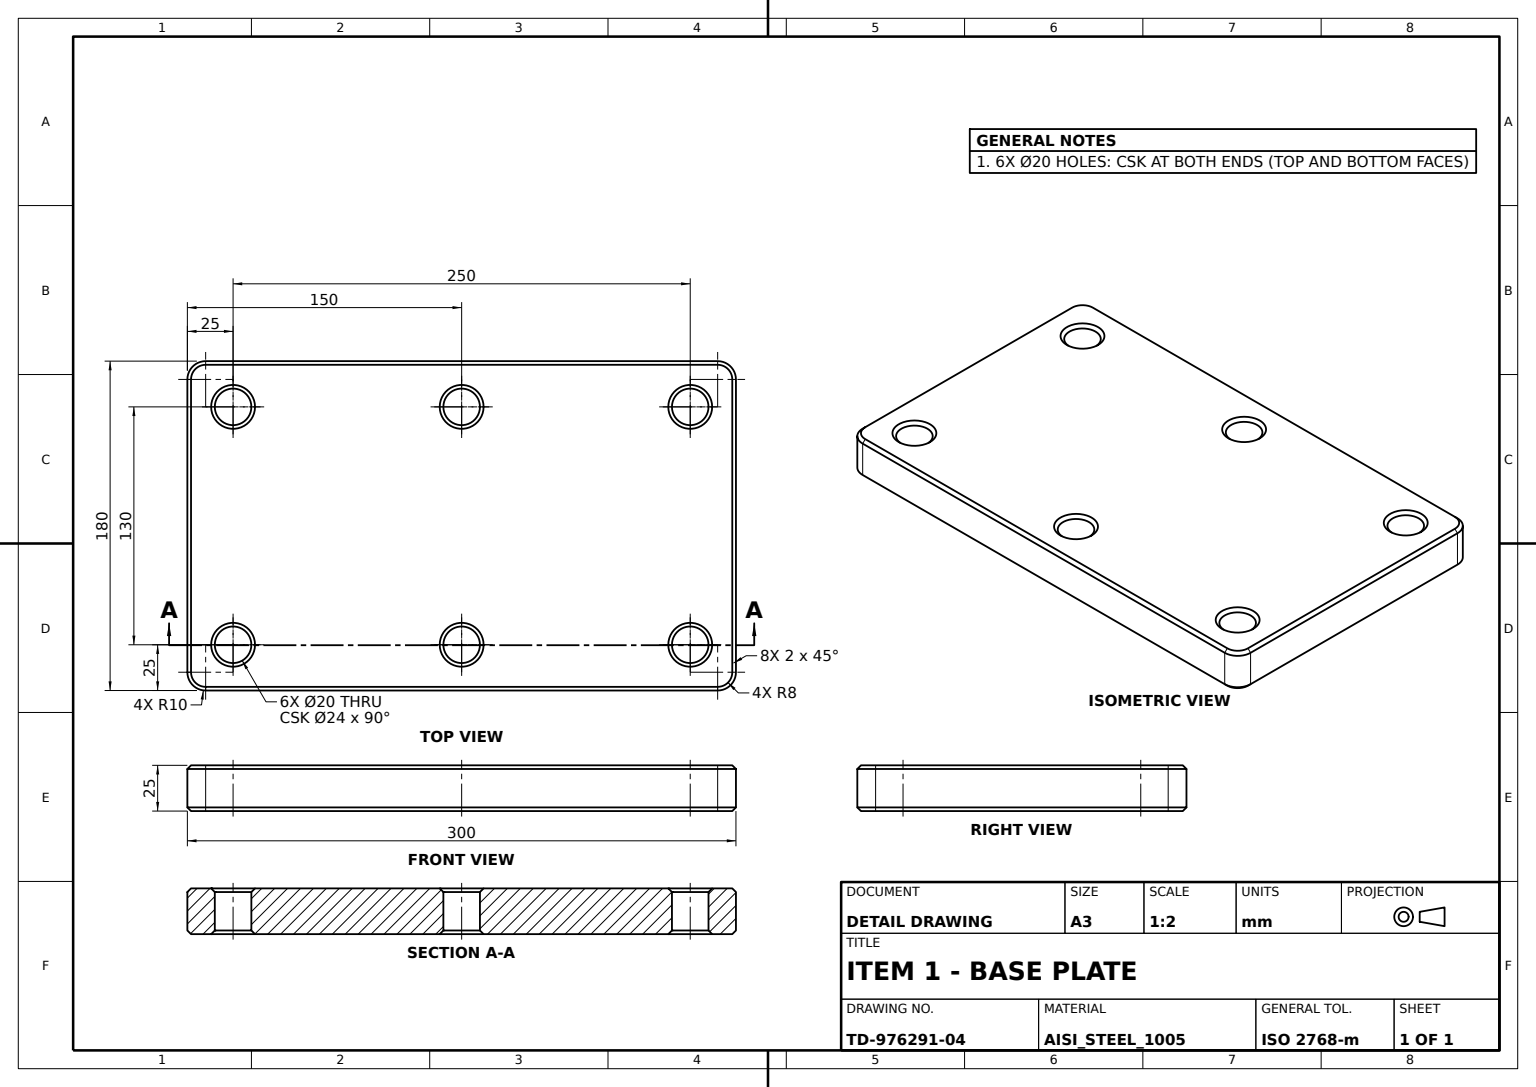
ISO-10303-21;
HEADER;
FILE_DESCRIPTION((''),'2;1');
FILE_NAME('','',(''),(''),'','','');
FILE_SCHEMA(('AUTOMOTIVE_DESIGN'));
ENDSEC;
DATA;
#1=APPLICATION_CONTEXT('');
#2=PRODUCT_CONTEXT('',#1,'mechanical');
#3=PRODUCT('','','',(#2));
#4=PRODUCT_DEFINITION_FORMATION('','',#3);
#5=PRODUCT_DEFINITION_CONTEXT('',#1,'design');
#6=PRODUCT_DEFINITION('','',#4,#5);
#7=PRODUCT_DEFINITION_SHAPE('','',#6);
#8=(LENGTH_UNIT()NAMED_UNIT(*)SI_UNIT(.MILLI.,.METRE.));
#9=(NAMED_UNIT(*)PLANE_ANGLE_UNIT()SI_UNIT($,.RADIAN.));
#10=(NAMED_UNIT(*)SI_UNIT($,.STERADIAN.)SOLID_ANGLE_UNIT());
#11=UNCERTAINTY_MEASURE_WITH_UNIT(LENGTH_MEASURE(0.005),#8,'distance_accuracy_value','');
#12=(GEOMETRIC_REPRESENTATION_CONTEXT(3)GLOBAL_UNCERTAINTY_ASSIGNED_CONTEXT((#11))GLOBAL_UNIT_ASSIGNED_CONTEXT((#8,#9,#10))REPRESENTATION_CONTEXT('',''));
#13=CARTESIAN_POINT('',(135.,65.,23.));
#14=VERTEX_POINT('',#13);
#15=CARTESIAN_POINT('',(125.,65.,23.));
#16=DIRECTION('',(0.,0.,1.));
#17=DIRECTION('',(1.,0.,0.));
#18=AXIS2_PLACEMENT_3D('',#15,#16,#17);
#19=CIRCLE('',#18,10.);
#20=EDGE_CURVE('',#14,#14,#19,.T.);
#21=ORIENTED_EDGE('',*,*,#20,.T.);
#22=EDGE_LOOP('',(#21));
#23=FACE_BOUND('',#22,.T.);
#24=CARTESIAN_POINT('',(135.,65.,2.));
#25=VERTEX_POINT('',#24);
#26=CARTESIAN_POINT('',(125.,65.,2.));
#27=AXIS2_PLACEMENT_3D('',#26,#16,#17);
#28=CIRCLE('',#27,10.);
#29=EDGE_CURVE('',#25,#25,#28,.F.);
#30=ORIENTED_EDGE('',*,*,#29,.T.);
#31=EDGE_LOOP('',(#30));
#32=FACE_BOUND('',#31,.T.);
#33=CARTESIAN_POINT('',(125.,65.,0.));
#34=AXIS2_PLACEMENT_3D('',#33,#16,#17);
#35=CYLINDRICAL_SURFACE('',#34,10.);
#36=ADVANCED_FACE('',(#23,#32),#35,.F.);
#37=CARTESIAN_POINT('',(-150.,80.,23.));
#38=VERTEX_POINT('',#37);
#39=CARTESIAN_POINT('',(-150.,80.,2.));
#40=VERTEX_POINT('',#39);
#41=CARTESIAN_POINT('',(-150.,80.,25.));
#42=DIRECTION('',(0.,0.,-1.));
#43=VECTOR('',#42,1000.);
#44=LINE('',#41,#43);
#45=EDGE_CURVE('',#38,#40,#44,.T.);
#46=ORIENTED_EDGE('',*,*,#45,.T.);
#47=CARTESIAN_POINT('',(-150.,-80.,2.));
#48=VERTEX_POINT('',#47);
#49=DIRECTION('',(0.,-1.,0.));
#50=VECTOR('',#49,1000.);
#51=LINE('',#39,#50);
#52=EDGE_CURVE('',#40,#48,#51,.T.);
#53=ORIENTED_EDGE('',*,*,#52,.T.);
#54=CARTESIAN_POINT('',(-150.,-80.,23.));
#55=VERTEX_POINT('',#54);
#56=CARTESIAN_POINT('',(-150.,-80.,25.));
#57=LINE('',#56,#43);
#58=EDGE_CURVE('',#55,#48,#57,.T.);
#59=ORIENTED_EDGE('',*,*,#58,.F.);
#60=DIRECTION('',(0.,1.,0.));
#61=VECTOR('',#60,1000.);
#62=LINE('',#37,#61);
#63=EDGE_CURVE('',#55,#38,#62,.T.);
#64=ORIENTED_EDGE('',*,*,#63,.T.);
#65=EDGE_LOOP('',(#46,#53,#59,#64));
#66=FACE_BOUND('',#65,.T.);
#67=AXIS2_PLACEMENT_3D('',#41,#17,#60);
#68=PLANE('',#67);
#69=ADVANCED_FACE('',(#66),#68,.F.);
#70=CARTESIAN_POINT('',(140.,90.,23.));
#71=VERTEX_POINT('',#70);
#72=CARTESIAN_POINT('',(140.,88.,25.));
#73=VERTEX_POINT('',#72);
#74=DIRECTION('',(0.,-0.707106781,0.707106781));
#75=VECTOR('',#74,1000.);
#76=LINE('',#70,#75);
#77=EDGE_CURVE('',#71,#73,#76,.T.);
#78=ORIENTED_EDGE('',*,*,#77,.F.);
#79=CARTESIAN_POINT('',(-140.,90.,23.));
#80=VERTEX_POINT('',#79);
#81=VECTOR('',#17,1000.);
#82=LINE('',#70,#81);
#83=EDGE_CURVE('',#80,#71,#82,.T.);
#84=ORIENTED_EDGE('',*,*,#83,.F.);
#85=CARTESIAN_POINT('',(-140.,88.,25.));
#86=VERTEX_POINT('',#85);
#87=LINE('',#79,#75);
#88=EDGE_CURVE('',#80,#86,#87,.T.);
#89=ORIENTED_EDGE('',*,*,#88,.T.);
#90=DIRECTION('',(-1.,0.,0.));
#91=VECTOR('',#90,1000.);
#92=LINE('',#85,#91);
#93=EDGE_CURVE('',#73,#86,#92,.T.);
#94=ORIENTED_EDGE('',*,*,#93,.F.);
#95=EDGE_LOOP('',(#78,#84,#89,#94));
#96=FACE_BOUND('',#95,.T.);
#97=DIRECTION('',(0.,0.707106781,0.707106781));
#98=AXIS2_PLACEMENT_3D('',#85,#97,#17);
#99=PLANE('',#98);
#100=ADVANCED_FACE('',(#96),#99,.T.);
#101=CARTESIAN_POINT('',(140.,-88.,0.));
#102=VERTEX_POINT('',#101);
#103=CARTESIAN_POINT('',(-140.,-88.,0.));
#104=VERTEX_POINT('',#103);
#105=LINE('',#103,#91);
#106=EDGE_CURVE('',#102,#104,#105,.T.);
#107=ORIENTED_EDGE('',*,*,#106,.F.);
#108=CARTESIAN_POINT('',(140.,-90.,2.));
#109=VERTEX_POINT('',#108);
#110=DIRECTION('',(0.,0.707106781,-0.707106781));
#111=VECTOR('',#110,1000.);
#112=LINE('',#108,#111);
#113=EDGE_CURVE('',#109,#102,#112,.T.);
#114=ORIENTED_EDGE('',*,*,#113,.F.);
#115=CARTESIAN_POINT('',(-140.,-90.,2.));
#116=VERTEX_POINT('',#115);
#117=LINE('',#115,#81);
#118=EDGE_CURVE('',#116,#109,#117,.T.);
#119=ORIENTED_EDGE('',*,*,#118,.F.);
#120=LINE('',#115,#111);
#121=EDGE_CURVE('',#116,#104,#120,.T.);
#122=ORIENTED_EDGE('',*,*,#121,.T.);
#123=EDGE_LOOP('',(#107,#114,#119,#122));
#124=FACE_BOUND('',#123,.T.);
#125=AXIS2_PLACEMENT_3D('',#115,#97,#17);
#126=PLANE('',#125);
#127=ADVANCED_FACE('',(#124),#126,.F.);
#128=CARTESIAN_POINT('',(135.,-65.,23.));
#129=VERTEX_POINT('',#128);
#130=CARTESIAN_POINT('',(125.,-65.,23.));
#131=AXIS2_PLACEMENT_3D('',#130,#16,#17);
#132=CIRCLE('',#131,10.);
#133=EDGE_CURVE('',#129,#129,#132,.T.);
#134=ORIENTED_EDGE('',*,*,#133,.T.);
#135=EDGE_LOOP('',(#134));
#136=FACE_BOUND('',#135,.T.);
#137=CARTESIAN_POINT('',(135.,-65.,2.));
#138=VERTEX_POINT('',#137);
#139=CARTESIAN_POINT('',(125.,-65.,2.));
#140=AXIS2_PLACEMENT_3D('',#139,#16,#17);
#141=CIRCLE('',#140,10.);
#142=EDGE_CURVE('',#138,#138,#141,.F.);
#143=ORIENTED_EDGE('',*,*,#142,.T.);
#144=EDGE_LOOP('',(#143));
#145=FACE_BOUND('',#144,.T.);
#146=CARTESIAN_POINT('',(125.,-65.,0.));
#147=AXIS2_PLACEMENT_3D('',#146,#16,#17);
#148=CYLINDRICAL_SURFACE('',#147,10.);
#149=ADVANCED_FACE('',(#136,#145),#148,.F.);
#150=CARTESIAN_POINT('',(-113.,65.,0.));
#151=VERTEX_POINT('',#150);
#152=CARTESIAN_POINT('',(-125.,65.,0.));
#153=AXIS2_PLACEMENT_3D('',#152,#16,#17);
#154=CIRCLE('',#153,12.);
#155=EDGE_CURVE('',#151,#151,#154,.T.);
#156=ORIENTED_EDGE('',*,*,#155,.F.);
#157=EDGE_LOOP('',(#156));
#158=FACE_BOUND('',#157,.T.);
#159=CARTESIAN_POINT('',(-115.,65.,2.));
#160=VERTEX_POINT('',#159);
#161=CARTESIAN_POINT('',(-125.,65.,2.));
#162=AXIS2_PLACEMENT_3D('',#161,#16,#17);
#163=CIRCLE('',#162,10.);
#164=EDGE_CURVE('',#160,#160,#163,.F.);
#165=ORIENTED_EDGE('',*,*,#164,.F.);
#166=EDGE_LOOP('',(#165));
#167=FACE_BOUND('',#166,.T.);
#168=AXIS2_PLACEMENT_3D('',#152,#42,#90);
#169=CONICAL_SURFACE('',#168,12.,0.785398163);
#170=ADVANCED_FACE('',(#158,#167),#169,.F.);
#171=CARTESIAN_POINT('',(-148.,80.,0.));
#172=VERTEX_POINT('',#171);
#173=DIRECTION('',(0.707106781,0.,-0.707106781));
#174=VECTOR('',#173,1000.);
#175=LINE('',#39,#174);
#176=EDGE_CURVE('',#40,#172,#175,.T.);
#177=ORIENTED_EDGE('',*,*,#176,.F.);
#178=CARTESIAN_POINT('',(-140.,90.,2.));
#179=VERTEX_POINT('',#178);
#180=CARTESIAN_POINT('',(-140.,80.,2.));
#181=AXIS2_PLACEMENT_3D('',#180,#16,#17);
#182=CIRCLE('',#181,10.);
#183=EDGE_CURVE('',#179,#40,#182,.T.);
#184=ORIENTED_EDGE('',*,*,#183,.F.);
#185=CARTESIAN_POINT('',(-140.,88.,0.));
#186=VERTEX_POINT('',#185);
#187=VECTOR('',#97,1000.);
#188=LINE('',#185,#187);
#189=EDGE_CURVE('',#186,#179,#188,.T.);
#190=ORIENTED_EDGE('',*,*,#189,.F.);
#191=CARTESIAN_POINT('',(-140.,80.,0.));
#192=AXIS2_PLACEMENT_3D('',#191,#16,#17);
#193=CIRCLE('',#192,8.);
#194=EDGE_CURVE('',#172,#186,#193,.F.);
#195=ORIENTED_EDGE('',*,*,#194,.F.);
#196=EDGE_LOOP('',(#177,#184,#190,#195));
#197=FACE_BOUND('',#196,.T.);
#198=CONICAL_SURFACE('',#181,10.,0.785398163);
#199=ADVANCED_FACE('',(#197),#198,.T.);
#200=CARTESIAN_POINT('',(10.,-65.,23.));
#201=VERTEX_POINT('',#200);
#202=CARTESIAN_POINT('',(0.,-65.,23.));
#203=AXIS2_PLACEMENT_3D('',#202,#16,#17);
#204=CIRCLE('',#203,10.);
#205=EDGE_CURVE('',#201,#201,#204,.T.);
#206=ORIENTED_EDGE('',*,*,#205,.T.);
#207=EDGE_LOOP('',(#206));
#208=FACE_BOUND('',#207,.T.);
#209=CARTESIAN_POINT('',(10.,-65.,2.));
#210=VERTEX_POINT('',#209);
#211=CARTESIAN_POINT('',(0.,-65.,2.));
#212=AXIS2_PLACEMENT_3D('',#211,#16,#17);
#213=CIRCLE('',#212,10.);
#214=EDGE_CURVE('',#210,#210,#213,.F.);
#215=ORIENTED_EDGE('',*,*,#214,.T.);
#216=EDGE_LOOP('',(#215));
#217=FACE_BOUND('',#216,.T.);
#218=CARTESIAN_POINT('',(0.,-65.,0.));
#219=AXIS2_PLACEMENT_3D('',#218,#16,#17);
#220=CYLINDRICAL_SURFACE('',#219,10.);
#221=ADVANCED_FACE('',(#208,#217),#220,.F.);
#222=CARTESIAN_POINT('',(12.,65.,0.));
#223=VERTEX_POINT('',#222);
#224=CARTESIAN_POINT('',(0.,65.,0.));
#225=AXIS2_PLACEMENT_3D('',#224,#16,#17);
#226=CIRCLE('',#225,12.);
#227=EDGE_CURVE('',#223,#223,#226,.T.);
#228=ORIENTED_EDGE('',*,*,#227,.F.);
#229=EDGE_LOOP('',(#228));
#230=FACE_BOUND('',#229,.T.);
#231=CARTESIAN_POINT('',(10.,65.,2.));
#232=VERTEX_POINT('',#231);
#233=CARTESIAN_POINT('',(0.,65.,2.));
#234=AXIS2_PLACEMENT_3D('',#233,#16,#17);
#235=CIRCLE('',#234,10.);
#236=EDGE_CURVE('',#232,#232,#235,.F.);
#237=ORIENTED_EDGE('',*,*,#236,.F.);
#238=EDGE_LOOP('',(#237));
#239=FACE_BOUND('',#238,.T.);
#240=AXIS2_PLACEMENT_3D('',#224,#42,#90);
#241=CONICAL_SURFACE('',#240,12.,0.785398163);
#242=ADVANCED_FACE('',(#230,#239),#241,.F.);
#243=CARTESIAN_POINT('',(-115.,-65.,2.));
#244=VERTEX_POINT('',#243);
#245=CARTESIAN_POINT('',(-125.,-65.,2.));
#246=AXIS2_PLACEMENT_3D('',#245,#16,#17);
#247=CIRCLE('',#246,10.);
#248=EDGE_CURVE('',#244,#244,#247,.F.);
#249=ORIENTED_EDGE('',*,*,#248,.F.);
#250=EDGE_LOOP('',(#249));
#251=FACE_BOUND('',#250,.T.);
#252=CARTESIAN_POINT('',(-113.,-65.,0.));
#253=VERTEX_POINT('',#252);
#254=CARTESIAN_POINT('',(-125.,-65.,0.));
#255=AXIS2_PLACEMENT_3D('',#254,#16,#17);
#256=CIRCLE('',#255,12.);
#257=EDGE_CURVE('',#253,#253,#256,.T.);
#258=ORIENTED_EDGE('',*,*,#257,.F.);
#259=EDGE_LOOP('',(#258));
#260=FACE_BOUND('',#259,.T.);
#261=AXIS2_PLACEMENT_3D('',#254,#42,#90);
#262=CONICAL_SURFACE('',#261,12.,0.785398163);
#263=ADVANCED_FACE('',(#251,#260),#262,.F.);
#264=CARTESIAN_POINT('',(137.,-65.,25.));
#265=VERTEX_POINT('',#264);
#266=CARTESIAN_POINT('',(125.,-65.,25.));
#267=AXIS2_PLACEMENT_3D('',#266,#16,#17);
#268=CIRCLE('',#267,12.);
#269=EDGE_CURVE('',#265,#265,#268,.F.);
#270=ORIENTED_EDGE('',*,*,#269,.F.);
#271=EDGE_LOOP('',(#270));
#272=FACE_BOUND('',#271,.T.);
#273=ORIENTED_EDGE('',*,*,#133,.F.);
#274=EDGE_LOOP('',(#273));
#275=FACE_BOUND('',#274,.T.);
#276=CONICAL_SURFACE('',#131,10.,0.785398163);
#277=ADVANCED_FACE('',(#272,#275),#276,.F.);
#278=CARTESIAN_POINT('',(-140.,-80.,2.));
#279=AXIS2_PLACEMENT_3D('',#278,#16,#17);
#280=CIRCLE('',#279,10.);
#281=EDGE_CURVE('',#48,#116,#280,.T.);
#282=ORIENTED_EDGE('',*,*,#281,.F.);
#283=CARTESIAN_POINT('',(-148.,-80.,0.));
#284=VERTEX_POINT('',#283);
#285=LINE('',#47,#174);
#286=EDGE_CURVE('',#48,#284,#285,.T.);
#287=ORIENTED_EDGE('',*,*,#286,.T.);
#288=CARTESIAN_POINT('',(-140.,-80.,0.));
#289=AXIS2_PLACEMENT_3D('',#288,#16,#17);
#290=CIRCLE('',#289,8.);
#291=EDGE_CURVE('',#104,#284,#290,.F.);
#292=ORIENTED_EDGE('',*,*,#291,.F.);
#293=ORIENTED_EDGE('',*,*,#121,.F.);
#294=EDGE_LOOP('',(#282,#287,#292,#293));
#295=FACE_BOUND('',#294,.T.);
#296=CONICAL_SURFACE('',#279,10.,0.785398163);
#297=ADVANCED_FACE('',(#295),#296,.T.);
#298=CARTESIAN_POINT('',(150.,80.,23.));
#299=VERTEX_POINT('',#298);
#300=CARTESIAN_POINT('',(140.,80.,23.));
#301=AXIS2_PLACEMENT_3D('',#300,#16,#17);
#302=CIRCLE('',#301,10.);
#303=EDGE_CURVE('',#71,#299,#302,.F.);
#304=ORIENTED_EDGE('',*,*,#303,.T.);
#305=CARTESIAN_POINT('',(150.,80.,2.));
#306=VERTEX_POINT('',#305);
#307=CARTESIAN_POINT('',(150.,80.,25.));
#308=LINE('',#307,#43);
#309=EDGE_CURVE('',#299,#306,#308,.T.);
#310=ORIENTED_EDGE('',*,*,#309,.T.);
#311=CARTESIAN_POINT('',(140.,90.,2.));
#312=VERTEX_POINT('',#311);
#313=CARTESIAN_POINT('',(140.,80.,2.));
#314=AXIS2_PLACEMENT_3D('',#313,#16,#17);
#315=CIRCLE('',#314,10.);
#316=EDGE_CURVE('',#306,#312,#315,.T.);
#317=ORIENTED_EDGE('',*,*,#316,.T.);
#318=CARTESIAN_POINT('',(140.,90.,25.));
#319=LINE('',#318,#43);
#320=EDGE_CURVE('',#71,#312,#319,.T.);
#321=ORIENTED_EDGE('',*,*,#320,.F.);
#322=EDGE_LOOP('',(#304,#310,#317,#321));
#323=FACE_BOUND('',#322,.T.);
#324=CARTESIAN_POINT('',(140.,80.,25.));
#325=AXIS2_PLACEMENT_3D('',#324,#42,#90);
#326=CYLINDRICAL_SURFACE('',#325,10.);
#327=ADVANCED_FACE('',(#323),#326,.T.);
#328=ORIENTED_EDGE('',*,*,#63,.F.);
#329=CARTESIAN_POINT('',(-148.,-80.,25.));
#330=VERTEX_POINT('',#329);
#331=DIRECTION('',(-0.707106781,0.,-0.707106781));
#332=VECTOR('',#331,1000.);
#333=LINE('',#329,#332);
#334=EDGE_CURVE('',#330,#55,#333,.T.);
#335=ORIENTED_EDGE('',*,*,#334,.F.);
#336=CARTESIAN_POINT('',(-148.,80.,25.));
#337=VERTEX_POINT('',#336);
#338=LINE('',#329,#50);
#339=EDGE_CURVE('',#337,#330,#338,.T.);
#340=ORIENTED_EDGE('',*,*,#339,.F.);
#341=LINE('',#336,#332);
#342=EDGE_CURVE('',#337,#38,#341,.T.);
#343=ORIENTED_EDGE('',*,*,#342,.T.);
#344=EDGE_LOOP('',(#328,#335,#340,#343));
#345=FACE_BOUND('',#344,.T.);
#346=DIRECTION('',(-0.707106781,0.,0.707106781));
#347=AXIS2_PLACEMENT_3D('',#329,#346,#60);
#348=PLANE('',#347);
#349=ADVANCED_FACE('',(#345),#348,.T.);
#350=CARTESIAN_POINT('',(12.,65.,25.));
#351=VERTEX_POINT('',#350);
#352=CARTESIAN_POINT('',(0.,65.,25.));
#353=AXIS2_PLACEMENT_3D('',#352,#16,#17);
#354=CIRCLE('',#353,12.);
#355=EDGE_CURVE('',#351,#351,#354,.F.);
#356=ORIENTED_EDGE('',*,*,#355,.F.);
#357=EDGE_LOOP('',(#356));
#358=FACE_BOUND('',#357,.T.);
#359=CARTESIAN_POINT('',(10.,65.,23.));
#360=VERTEX_POINT('',#359);
#361=CARTESIAN_POINT('',(0.,65.,23.));
#362=AXIS2_PLACEMENT_3D('',#361,#16,#17);
#363=CIRCLE('',#362,10.);
#364=EDGE_CURVE('',#360,#360,#363,.T.);
#365=ORIENTED_EDGE('',*,*,#364,.F.);
#366=EDGE_LOOP('',(#365));
#367=FACE_BOUND('',#366,.T.);
#368=CONICAL_SURFACE('',#362,10.,0.785398163);
#369=ADVANCED_FACE('',(#358,#367),#368,.F.);
#370=ORIENTED_EDGE('',*,*,#248,.T.);
#371=EDGE_LOOP('',(#370));
#372=FACE_BOUND('',#371,.T.);
#373=CARTESIAN_POINT('',(-115.,-65.,23.));
#374=VERTEX_POINT('',#373);
#375=CARTESIAN_POINT('',(-125.,-65.,23.));
#376=AXIS2_PLACEMENT_3D('',#375,#16,#17);
#377=CIRCLE('',#376,10.);
#378=EDGE_CURVE('',#374,#374,#377,.T.);
#379=ORIENTED_EDGE('',*,*,#378,.T.);
#380=EDGE_LOOP('',(#379));
#381=FACE_BOUND('',#380,.T.);
#382=CYLINDRICAL_SURFACE('',#255,10.);
#383=ADVANCED_FACE('',(#372,#381),#382,.F.);
#384=ORIENTED_EDGE('',*,*,#214,.F.);
#385=EDGE_LOOP('',(#384));
#386=FACE_BOUND('',#385,.T.);
#387=CARTESIAN_POINT('',(12.,-65.,0.));
#388=VERTEX_POINT('',#387);
#389=CIRCLE('',#219,12.);
#390=EDGE_CURVE('',#388,#388,#389,.T.);
#391=ORIENTED_EDGE('',*,*,#390,.F.);
#392=EDGE_LOOP('',(#391));
#393=FACE_BOUND('',#392,.T.);
#394=AXIS2_PLACEMENT_3D('',#218,#42,#90);
#395=CONICAL_SURFACE('',#394,12.,0.785398163);
#396=ADVANCED_FACE('',(#386,#393),#395,.F.);
#397=CARTESIAN_POINT('',(148.,-80.,0.));
#398=VERTEX_POINT('',#397);
#399=CARTESIAN_POINT('',(150.,-80.,2.));
#400=VERTEX_POINT('',#399);
#401=DIRECTION('',(0.707106781,0.,0.707106781));
#402=VECTOR('',#401,1000.);
#403=LINE('',#397,#402);
#404=EDGE_CURVE('',#398,#400,#403,.T.);
#405=ORIENTED_EDGE('',*,*,#404,.F.);
#406=CARTESIAN_POINT('',(148.,80.,0.));
#407=VERTEX_POINT('',#406);
#408=LINE('',#397,#50);
#409=EDGE_CURVE('',#407,#398,#408,.T.);
#410=ORIENTED_EDGE('',*,*,#409,.F.);
#411=LINE('',#406,#402);
#412=EDGE_CURVE('',#407,#306,#411,.T.);
#413=ORIENTED_EDGE('',*,*,#412,.T.);
#414=LINE('',#399,#61);
#415=EDGE_CURVE('',#400,#306,#414,.T.);
#416=ORIENTED_EDGE('',*,*,#415,.F.);
#417=EDGE_LOOP('',(#405,#410,#413,#416));
#418=FACE_BOUND('',#417,.T.);
#419=AXIS2_PLACEMENT_3D('',#399,#346,#60);
#420=PLANE('',#419);
#421=ADVANCED_FACE('',(#418),#420,.F.);
#422=CARTESIAN_POINT('',(140.,-80.,2.));
#423=AXIS2_PLACEMENT_3D('',#422,#16,#17);
#424=CIRCLE('',#423,10.);
#425=EDGE_CURVE('',#109,#400,#424,.T.);
#426=ORIENTED_EDGE('',*,*,#425,.F.);
#427=ORIENTED_EDGE('',*,*,#113,.T.);
#428=CARTESIAN_POINT('',(140.,-80.,0.));
#429=AXIS2_PLACEMENT_3D('',#428,#16,#17);
#430=CIRCLE('',#429,8.);
#431=EDGE_CURVE('',#398,#102,#430,.F.);
#432=ORIENTED_EDGE('',*,*,#431,.F.);
#433=ORIENTED_EDGE('',*,*,#404,.T.);
#434=EDGE_LOOP('',(#426,#427,#432,#433));
#435=FACE_BOUND('',#434,.T.);
#436=CONICAL_SURFACE('',#423,10.,0.785398163);
#437=ADVANCED_FACE('',(#435),#436,.T.);
#438=ORIENTED_EDGE('',*,*,#88,.F.);
#439=CARTESIAN_POINT('',(-140.,80.,23.));
#440=AXIS2_PLACEMENT_3D('',#439,#16,#17);
#441=CIRCLE('',#440,10.);
#442=EDGE_CURVE('',#38,#80,#441,.F.);
#443=ORIENTED_EDGE('',*,*,#442,.F.);
#444=ORIENTED_EDGE('',*,*,#342,.F.);
#445=CARTESIAN_POINT('',(-140.,80.,25.));
#446=AXIS2_PLACEMENT_3D('',#445,#16,#17);
#447=CIRCLE('',#446,8.);
#448=EDGE_CURVE('',#86,#337,#447,.T.);
#449=ORIENTED_EDGE('',*,*,#448,.F.);
#450=EDGE_LOOP('',(#438,#443,#444,#449));
#451=FACE_BOUND('',#450,.T.);
#452=AXIS2_PLACEMENT_3D('',#445,#42,#90);
#453=CONICAL_SURFACE('',#452,8.,0.785398163);
#454=ADVANCED_FACE('',(#451),#453,.T.);
#455=CARTESIAN_POINT('',(-140.,90.,25.));
#456=LINE('',#455,#43);
#457=EDGE_CURVE('',#80,#179,#456,.T.);
#458=ORIENTED_EDGE('',*,*,#457,.T.);
#459=ORIENTED_EDGE('',*,*,#183,.T.);
#460=ORIENTED_EDGE('',*,*,#45,.F.);
#461=ORIENTED_EDGE('',*,*,#442,.T.);
#462=EDGE_LOOP('',(#458,#459,#460,#461));
#463=FACE_BOUND('',#462,.T.);
#464=CYLINDRICAL_SURFACE('',#452,10.);
#465=ADVANCED_FACE('',(#463),#464,.T.);
#466=ORIENTED_EDGE('',*,*,#425,.T.);
#467=CARTESIAN_POINT('',(150.,-80.,23.));
#468=VERTEX_POINT('',#467);
#469=CARTESIAN_POINT('',(150.,-80.,25.));
#470=LINE('',#469,#43);
#471=EDGE_CURVE('',#468,#400,#470,.T.);
#472=ORIENTED_EDGE('',*,*,#471,.F.);
#473=CARTESIAN_POINT('',(140.,-90.,23.));
#474=VERTEX_POINT('',#473);
#475=CARTESIAN_POINT('',(140.,-80.,23.));
#476=AXIS2_PLACEMENT_3D('',#475,#16,#17);
#477=CIRCLE('',#476,10.);
#478=EDGE_CURVE('',#468,#474,#477,.F.);
#479=ORIENTED_EDGE('',*,*,#478,.T.);
#480=CARTESIAN_POINT('',(140.,-90.,25.));
#481=LINE('',#480,#43);
#482=EDGE_CURVE('',#474,#109,#481,.T.);
#483=ORIENTED_EDGE('',*,*,#482,.T.);
#484=EDGE_LOOP('',(#466,#472,#479,#483));
#485=FACE_BOUND('',#484,.T.);
#486=CARTESIAN_POINT('',(140.,-80.,25.));
#487=AXIS2_PLACEMENT_3D('',#486,#42,#90);
#488=CYLINDRICAL_SURFACE('',#487,10.);
#489=ADVANCED_FACE('',(#485),#488,.T.);
#490=ORIENTED_EDGE('',*,*,#355,.T.);
#491=EDGE_LOOP('',(#490));
#492=FACE_BOUND('',#491,.T.);
#493=CARTESIAN_POINT('',(-140.,-88.,25.));
#494=VERTEX_POINT('',#493);
#495=CARTESIAN_POINT('',(-140.,-80.,25.));
#496=AXIS2_PLACEMENT_3D('',#495,#16,#17);
#497=CIRCLE('',#496,8.);
#498=EDGE_CURVE('',#330,#494,#497,.T.);
#499=ORIENTED_EDGE('',*,*,#498,.T.);
#500=CARTESIAN_POINT('',(140.,-88.,25.));
#501=VERTEX_POINT('',#500);
#502=LINE('',#500,#81);
#503=EDGE_CURVE('',#494,#501,#502,.T.);
#504=ORIENTED_EDGE('',*,*,#503,.T.);
#505=CARTESIAN_POINT('',(148.,-80.,25.));
#506=VERTEX_POINT('',#505);
#507=AXIS2_PLACEMENT_3D('',#486,#16,#17);
#508=CIRCLE('',#507,8.);
#509=EDGE_CURVE('',#501,#506,#508,.T.);
#510=ORIENTED_EDGE('',*,*,#509,.T.);
#511=CARTESIAN_POINT('',(148.,80.,25.));
#512=VERTEX_POINT('',#511);
#513=LINE('',#511,#61);
#514=EDGE_CURVE('',#506,#512,#513,.T.);
#515=ORIENTED_EDGE('',*,*,#514,.T.);
#516=AXIS2_PLACEMENT_3D('',#324,#16,#17);
#517=CIRCLE('',#516,8.);
#518=EDGE_CURVE('',#512,#73,#517,.T.);
#519=ORIENTED_EDGE('',*,*,#518,.T.);
#520=ORIENTED_EDGE('',*,*,#93,.T.);
#521=ORIENTED_EDGE('',*,*,#448,.T.);
#522=ORIENTED_EDGE('',*,*,#339,.T.);
#523=EDGE_LOOP('',(#499,#504,#510,#515,#519,#520,#521,#522));
#524=FACE_BOUND('',#523,.T.);
#525=CARTESIAN_POINT('',(137.,65.,25.));
#526=VERTEX_POINT('',#525);
#527=CARTESIAN_POINT('',(125.,65.,25.));
#528=AXIS2_PLACEMENT_3D('',#527,#16,#17);
#529=CIRCLE('',#528,12.);
#530=EDGE_CURVE('',#526,#526,#529,.F.);
#531=ORIENTED_EDGE('',*,*,#530,.T.);
#532=EDGE_LOOP('',(#531));
#533=FACE_BOUND('',#532,.T.);
#534=CARTESIAN_POINT('',(-113.,-65.,25.));
#535=VERTEX_POINT('',#534);
#536=CARTESIAN_POINT('',(-125.,-65.,25.));
#537=AXIS2_PLACEMENT_3D('',#536,#16,#17);
#538=CIRCLE('',#537,12.);
#539=EDGE_CURVE('',#535,#535,#538,.F.);
#540=ORIENTED_EDGE('',*,*,#539,.T.);
#541=EDGE_LOOP('',(#540));
#542=FACE_BOUND('',#541,.T.);
#543=CARTESIAN_POINT('',(-113.,65.,25.));
#544=VERTEX_POINT('',#543);
#545=CARTESIAN_POINT('',(-125.,65.,25.));
#546=AXIS2_PLACEMENT_3D('',#545,#16,#17);
#547=CIRCLE('',#546,12.);
#548=EDGE_CURVE('',#544,#544,#547,.F.);
#549=ORIENTED_EDGE('',*,*,#548,.T.);
#550=EDGE_LOOP('',(#549));
#551=FACE_BOUND('',#550,.T.);
#552=CARTESIAN_POINT('',(12.,-65.,25.));
#553=VERTEX_POINT('',#552);
#554=CARTESIAN_POINT('',(0.,-65.,25.));
#555=AXIS2_PLACEMENT_3D('',#554,#16,#17);
#556=CIRCLE('',#555,12.);
#557=EDGE_CURVE('',#553,#553,#556,.F.);
#558=ORIENTED_EDGE('',*,*,#557,.T.);
#559=EDGE_LOOP('',(#558));
#560=FACE_BOUND('',#559,.T.);
#561=ORIENTED_EDGE('',*,*,#269,.T.);
#562=EDGE_LOOP('',(#561));
#563=FACE_BOUND('',#562,.T.);
#564=PLANE('',#496);
#565=ADVANCED_FACE('',(#492,#524,#533,#542,#551,#560,#563),#564,.T.);
#566=LINE('',#467,#50);
#567=EDGE_CURVE('',#299,#468,#566,.T.);
#568=ORIENTED_EDGE('',*,*,#567,.F.);
#569=VECTOR('',#346,1000.);
#570=LINE('',#298,#569);
#571=EDGE_CURVE('',#299,#512,#570,.T.);
#572=ORIENTED_EDGE('',*,*,#571,.T.);
#573=ORIENTED_EDGE('',*,*,#514,.F.);
#574=LINE('',#467,#569);
#575=EDGE_CURVE('',#468,#506,#574,.T.);
#576=ORIENTED_EDGE('',*,*,#575,.F.);
#577=EDGE_LOOP('',(#568,#572,#573,#576));
#578=FACE_BOUND('',#577,.T.);
#579=AXIS2_PLACEMENT_3D('',#505,#401,#49);
#580=PLANE('',#579);
#581=ADVANCED_FACE('',(#578),#580,.T.);
#582=ORIENTED_EDGE('',*,*,#189,.T.);
#583=LINE('',#311,#91);
#584=EDGE_CURVE('',#312,#179,#583,.T.);
#585=ORIENTED_EDGE('',*,*,#584,.F.);
#586=CARTESIAN_POINT('',(140.,88.,0.));
#587=VERTEX_POINT('',#586);
#588=LINE('',#586,#187);
#589=EDGE_CURVE('',#587,#312,#588,.T.);
#590=ORIENTED_EDGE('',*,*,#589,.F.);
#591=LINE('',#185,#81);
#592=EDGE_CURVE('',#186,#587,#591,.T.);
#593=ORIENTED_EDGE('',*,*,#592,.F.);
#594=EDGE_LOOP('',(#582,#585,#590,#593));
#595=FACE_BOUND('',#594,.T.);
#596=AXIS2_PLACEMENT_3D('',#311,#74,#90);
#597=PLANE('',#596);
#598=ADVANCED_FACE('',(#595),#597,.F.);
#599=ORIENTED_EDGE('',*,*,#557,.F.);
#600=EDGE_LOOP('',(#599));
#601=FACE_BOUND('',#600,.T.);
#602=ORIENTED_EDGE('',*,*,#205,.F.);
#603=EDGE_LOOP('',(#602));
#604=FACE_BOUND('',#603,.T.);
#605=CONICAL_SURFACE('',#203,10.,0.785398163);
#606=ADVANCED_FACE('',(#601,#604),#605,.F.);
#607=ORIENTED_EDGE('',*,*,#530,.F.);
#608=EDGE_LOOP('',(#607));
#609=FACE_BOUND('',#608,.T.);
#610=ORIENTED_EDGE('',*,*,#20,.F.);
#611=EDGE_LOOP('',(#610));
#612=FACE_BOUND('',#611,.T.);
#613=CONICAL_SURFACE('',#18,10.,0.785398163);
#614=ADVANCED_FACE('',(#609,#612),#613,.F.);
#615=ORIENTED_EDGE('',*,*,#316,.F.);
#616=ORIENTED_EDGE('',*,*,#412,.F.);
#617=CARTESIAN_POINT('',(140.,80.,0.));
#618=AXIS2_PLACEMENT_3D('',#617,#16,#17);
#619=CIRCLE('',#618,8.);
#620=EDGE_CURVE('',#587,#407,#619,.F.);
#621=ORIENTED_EDGE('',*,*,#620,.F.);
#622=ORIENTED_EDGE('',*,*,#589,.T.);
#623=EDGE_LOOP('',(#615,#616,#621,#622));
#624=FACE_BOUND('',#623,.T.);
#625=CONICAL_SURFACE('',#314,10.,0.785398163);
#626=ADVANCED_FACE('',(#624),#625,.T.);
#627=ORIENTED_EDGE('',*,*,#548,.F.);
#628=EDGE_LOOP('',(#627));
#629=FACE_BOUND('',#628,.T.);
#630=CARTESIAN_POINT('',(-115.,65.,23.));
#631=VERTEX_POINT('',#630);
#632=CARTESIAN_POINT('',(-125.,65.,23.));
#633=AXIS2_PLACEMENT_3D('',#632,#16,#17);
#634=CIRCLE('',#633,10.);
#635=EDGE_CURVE('',#631,#631,#634,.T.);
#636=ORIENTED_EDGE('',*,*,#635,.F.);
#637=EDGE_LOOP('',(#636));
#638=FACE_BOUND('',#637,.T.);
#639=CONICAL_SURFACE('',#633,10.,0.785398163);
#640=ADVANCED_FACE('',(#629,#638),#639,.F.);
#641=ORIENTED_EDGE('',*,*,#539,.F.);
#642=EDGE_LOOP('',(#641));
#643=FACE_BOUND('',#642,.T.);
#644=ORIENTED_EDGE('',*,*,#378,.F.);
#645=EDGE_LOOP('',(#644));
#646=FACE_BOUND('',#645,.T.);
#647=CONICAL_SURFACE('',#376,10.,0.785398163);
#648=ADVANCED_FACE('',(#643,#646),#647,.F.);
#649=ORIENTED_EDGE('',*,*,#503,.F.);
#650=CARTESIAN_POINT('',(-140.,-90.,23.));
#651=VERTEX_POINT('',#650);
#652=DIRECTION('',(0.,-0.707106781,-0.707106781));
#653=VECTOR('',#652,1000.);
#654=LINE('',#493,#653);
#655=EDGE_CURVE('',#494,#651,#654,.T.);
#656=ORIENTED_EDGE('',*,*,#655,.T.);
#657=LINE('',#650,#91);
#658=EDGE_CURVE('',#474,#651,#657,.T.);
#659=ORIENTED_EDGE('',*,*,#658,.F.);
#660=LINE('',#500,#653);
#661=EDGE_CURVE('',#501,#474,#660,.T.);
#662=ORIENTED_EDGE('',*,*,#661,.F.);
#663=EDGE_LOOP('',(#649,#656,#659,#662));
#664=FACE_BOUND('',#663,.T.);
#665=AXIS2_PLACEMENT_3D('',#493,#74,#90);
#666=PLANE('',#665);
#667=ADVANCED_FACE('',(#664),#666,.T.);
#668=ORIENTED_EDGE('',*,*,#236,.T.);
#669=EDGE_LOOP('',(#668));
#670=FACE_BOUND('',#669,.T.);
#671=ORIENTED_EDGE('',*,*,#364,.T.);
#672=EDGE_LOOP('',(#671));
#673=FACE_BOUND('',#672,.T.);
#674=CYLINDRICAL_SURFACE('',#225,10.);
#675=ADVANCED_FACE('',(#670,#673),#674,.F.);
#676=ORIENTED_EDGE('',*,*,#575,.T.);
#677=ORIENTED_EDGE('',*,*,#509,.F.);
#678=ORIENTED_EDGE('',*,*,#661,.T.);
#679=ORIENTED_EDGE('',*,*,#478,.F.);
#680=EDGE_LOOP('',(#676,#677,#678,#679));
#681=FACE_BOUND('',#680,.T.);
#682=CONICAL_SURFACE('',#487,8.,0.785398163);
#683=ADVANCED_FACE('',(#681),#682,.T.);
#684=ORIENTED_EDGE('',*,*,#635,.T.);
#685=EDGE_LOOP('',(#684));
#686=FACE_BOUND('',#685,.T.);
#687=ORIENTED_EDGE('',*,*,#164,.T.);
#688=EDGE_LOOP('',(#687));
#689=FACE_BOUND('',#688,.T.);
#690=CYLINDRICAL_SURFACE('',#153,10.);
#691=ADVANCED_FACE('',(#686,#689),#690,.F.);
#692=ORIENTED_EDGE('',*,*,#303,.F.);
#693=ORIENTED_EDGE('',*,*,#77,.T.);
#694=ORIENTED_EDGE('',*,*,#518,.F.);
#695=ORIENTED_EDGE('',*,*,#571,.F.);
#696=EDGE_LOOP('',(#692,#693,#694,#695));
#697=FACE_BOUND('',#696,.T.);
#698=CONICAL_SURFACE('',#325,8.,0.785398163);
#699=ADVANCED_FACE('',(#697),#698,.T.);
#700=CARTESIAN_POINT('',(-140.,-80.,23.));
#701=AXIS2_PLACEMENT_3D('',#700,#16,#17);
#702=CIRCLE('',#701,10.);
#703=EDGE_CURVE('',#651,#55,#702,.F.);
#704=ORIENTED_EDGE('',*,*,#703,.T.);
#705=ORIENTED_EDGE('',*,*,#58,.T.);
#706=ORIENTED_EDGE('',*,*,#281,.T.);
#707=CARTESIAN_POINT('',(-140.,-90.,25.));
#708=LINE('',#707,#43);
#709=EDGE_CURVE('',#651,#116,#708,.T.);
#710=ORIENTED_EDGE('',*,*,#709,.F.);
#711=EDGE_LOOP('',(#704,#705,#706,#710));
#712=FACE_BOUND('',#711,.T.);
#713=AXIS2_PLACEMENT_3D('',#495,#42,#90);
#714=CYLINDRICAL_SURFACE('',#713,10.);
#715=ADVANCED_FACE('',(#712),#714,.T.);
#716=ORIENTED_EDGE('',*,*,#567,.T.);
#717=ORIENTED_EDGE('',*,*,#471,.T.);
#718=ORIENTED_EDGE('',*,*,#415,.T.);
#719=ORIENTED_EDGE('',*,*,#309,.F.);
#720=EDGE_LOOP('',(#716,#717,#718,#719));
#721=FACE_BOUND('',#720,.T.);
#722=AXIS2_PLACEMENT_3D('',#469,#90,#49);
#723=PLANE('',#722);
#724=ADVANCED_FACE('',(#721),#723,.F.);
#725=ORIENTED_EDGE('',*,*,#29,.F.);
#726=EDGE_LOOP('',(#725));
#727=FACE_BOUND('',#726,.T.);
#728=CARTESIAN_POINT('',(137.,65.,0.));
#729=VERTEX_POINT('',#728);
#730=CIRCLE('',#34,12.);
#731=EDGE_CURVE('',#729,#729,#730,.T.);
#732=ORIENTED_EDGE('',*,*,#731,.F.);
#733=EDGE_LOOP('',(#732));
#734=FACE_BOUND('',#733,.T.);
#735=AXIS2_PLACEMENT_3D('',#33,#42,#90);
#736=CONICAL_SURFACE('',#735,12.,0.785398163);
#737=ADVANCED_FACE('',(#727,#734),#736,.F.);
#738=ORIENTED_EDGE('',*,*,#658,.T.);
#739=ORIENTED_EDGE('',*,*,#709,.T.);
#740=ORIENTED_EDGE('',*,*,#118,.T.);
#741=ORIENTED_EDGE('',*,*,#482,.F.);
#742=EDGE_LOOP('',(#738,#739,#740,#741));
#743=FACE_BOUND('',#742,.T.);
#744=AXIS2_PLACEMENT_3D('',#707,#60,#16);
#745=PLANE('',#744);
#746=ADVANCED_FACE('',(#743),#745,.F.);
#747=ORIENTED_EDGE('',*,*,#176,.T.);
#748=LINE('',#283,#61);
#749=EDGE_CURVE('',#284,#172,#748,.T.);
#750=ORIENTED_EDGE('',*,*,#749,.F.);
#751=ORIENTED_EDGE('',*,*,#286,.F.);
#752=ORIENTED_EDGE('',*,*,#52,.F.);
#753=EDGE_LOOP('',(#747,#750,#751,#752));
#754=FACE_BOUND('',#753,.T.);
#755=AXIS2_PLACEMENT_3D('',#39,#401,#49);
#756=PLANE('',#755);
#757=ADVANCED_FACE('',(#754),#756,.F.);
#758=ORIENTED_EDGE('',*,*,#291,.T.);
#759=ORIENTED_EDGE('',*,*,#749,.T.);
#760=ORIENTED_EDGE('',*,*,#194,.T.);
#761=ORIENTED_EDGE('',*,*,#592,.T.);
#762=ORIENTED_EDGE('',*,*,#620,.T.);
#763=ORIENTED_EDGE('',*,*,#409,.T.);
#764=ORIENTED_EDGE('',*,*,#431,.T.);
#765=ORIENTED_EDGE('',*,*,#106,.T.);
#766=EDGE_LOOP('',(#758,#759,#760,#761,#762,#763,#764,#765));
#767=FACE_BOUND('',#766,.T.);
#768=ORIENTED_EDGE('',*,*,#155,.T.);
#769=EDGE_LOOP('',(#768));
#770=FACE_BOUND('',#769,.T.);
#771=ORIENTED_EDGE('',*,*,#227,.T.);
#772=EDGE_LOOP('',(#771));
#773=FACE_BOUND('',#772,.T.);
#774=ORIENTED_EDGE('',*,*,#257,.T.);
#775=EDGE_LOOP('',(#774));
#776=FACE_BOUND('',#775,.T.);
#777=ORIENTED_EDGE('',*,*,#390,.T.);
#778=EDGE_LOOP('',(#777));
#779=FACE_BOUND('',#778,.T.);
#780=ORIENTED_EDGE('',*,*,#731,.T.);
#781=EDGE_LOOP('',(#780));
#782=FACE_BOUND('',#781,.T.);
#783=CARTESIAN_POINT('',(137.,-65.,0.));
#784=VERTEX_POINT('',#783);
#785=CIRCLE('',#147,12.);
#786=EDGE_CURVE('',#784,#784,#785,.T.);
#787=ORIENTED_EDGE('',*,*,#786,.T.);
#788=EDGE_LOOP('',(#787));
#789=FACE_BOUND('',#788,.T.);
#790=PLANE('',#289);
#791=ADVANCED_FACE('',(#767,#770,#773,#776,#779,#782,#789),#790,.F.);
#792=ORIENTED_EDGE('',*,*,#584,.T.);
#793=ORIENTED_EDGE('',*,*,#457,.F.);
#794=ORIENTED_EDGE('',*,*,#83,.T.);
#795=ORIENTED_EDGE('',*,*,#320,.T.);
#796=EDGE_LOOP('',(#792,#793,#794,#795));
#797=FACE_BOUND('',#796,.T.);
#798=AXIS2_PLACEMENT_3D('',#318,#49,#17);
#799=PLANE('',#798);
#800=ADVANCED_FACE('',(#797),#799,.F.);
#801=ORIENTED_EDGE('',*,*,#142,.F.);
#802=EDGE_LOOP('',(#801));
#803=FACE_BOUND('',#802,.T.);
#804=ORIENTED_EDGE('',*,*,#786,.F.);
#805=EDGE_LOOP('',(#804));
#806=FACE_BOUND('',#805,.T.);
#807=AXIS2_PLACEMENT_3D('',#146,#42,#90);
#808=CONICAL_SURFACE('',#807,12.,0.785398163);
#809=ADVANCED_FACE('',(#803,#806),#808,.F.);
#810=ORIENTED_EDGE('',*,*,#655,.F.);
#811=ORIENTED_EDGE('',*,*,#498,.F.);
#812=ORIENTED_EDGE('',*,*,#334,.T.);
#813=ORIENTED_EDGE('',*,*,#703,.F.);
#814=EDGE_LOOP('',(#810,#811,#812,#813));
#815=FACE_BOUND('',#814,.T.);
#816=CONICAL_SURFACE('',#713,8.,0.785398163);
#817=ADVANCED_FACE('',(#815),#816,.T.);
#818=CLOSED_SHELL('',(#36,#69,#100,#127,#149,#170,#199,#221,#242,#263,#277,#297,#327,#349,#369,#383,#396,#421,#437,#454,#465,#489,#565,#581,#598,#606,#614,#626,#640,#648,#667,#675,#683,#691,#699,#715,#724,#737,#746,#757,#791,#800,#809,#817));
#819=MANIFOLD_SOLID_BREP('',#818);
#820=ADVANCED_BREP_SHAPE_REPRESENTATION('',(#819),#12);
#821=SHAPE_DEFINITION_REPRESENTATION(#7,#820);
ENDSEC;
END-ISO-10303-21;
